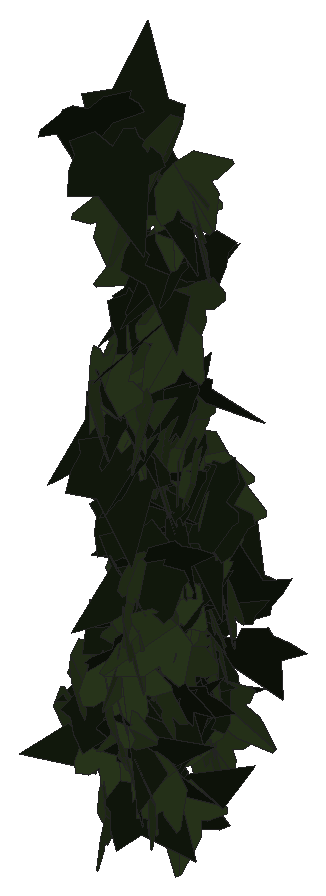
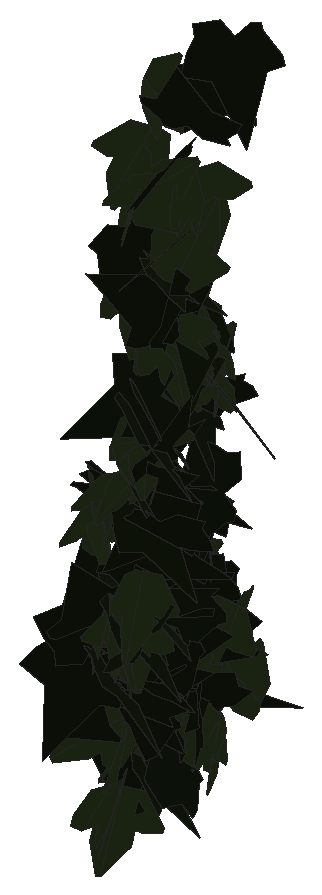
# SketchUp Ruby script. Lengths in inches.
U = 1.inch
M = Sketchup.active_model
def pt(a) = Geom::Point3d.new(a.map { |v| v * U })
def face(e, loops, mat)
  f = e.add_face(loops[0].map { |a| pt(a) })
  loops[1..].each { |l| e.add_face(l.map { |a| pt(a) }).erase! }
  f.material = f.back_material = mat if mat
  f
end
# faces: each face lists its corners as indices into pts; further lists are holes
def faces(e, pts, list, mat = nil) = list.each { |f| face(e, (f[0].is_a?(Array) ? f : [f]).map { |l| l.map { |i| pts[i] } }, mat) }
# xy, xz, yz: faces in a plane at the given z, y or x. An outline is a flat list of corners, or four numbers for a rectangle; further outlines are holes
def ring(l) = l.size == 4 ? [[l[0], l[1]], [l[2], l[1]], [l[2], l[3]], [l[0], l[3]]] : l.each_slice(2).to_a
def flat(e, list, mat, &to3) = list.each { |f| face(e, (f[0].is_a?(Array) ? f : [f]).map { |l| ring(l).map { |u, v| to3.(u, v) } }, mat) }
def xy(e, z, list, mat = nil) = flat(e, list, mat) { |x, y| [x, y, z] }
def xz(e, y, list, mat = nil) = flat(e, list, mat) { |x, z| [x, y, z] }
def yz(e, x, list, mat = nil) = flat(e, list, mat) { |y, z| [x, y, z] }
def lines(e, pts, list) = list.each { |a, b| e.add_line(pt(pts[a]), pt(pts[b])) }
# prism: a flat outline (further loops are holes) pulled along v
def prism(e, loops, v, mat = nil)
  f = face(e, loops, mat); d = Geom::Vector3d.new(v.map { |x| x * U })
  f.pushpull(f.normal.samedirection?(d) ? d.length : -d.length)
end
def box(e, o, s, mat = nil) = prism(e, [[o, [o[0] + s[0], o[1], o[2]], [o[0] + s[0], o[1] + s[1], o[2]], [o[0], o[1] + s[1], o[2]]]], [0, 0, s[2]], mat)
def at(x, y, z, deg = 0) = Geom::Transformation.translation(pt([x, y, z])) * Geom::Transformation.rotation(ORIGIN, Z_AXIS, deg.degrees)
def axes(o, x, y, z) = Geom::Transformation.new([*x, 0, *y, 0, *z, 0, *pt(o).to_a, 1])
def part(name) = M.definitions.add(name)
# library, detail: a bought-in or finely detailed component or shape, given as its bounding box
def library(name, o, s) = part(name).tap { |d| box(d.entities, o, s) }
def detail(e, o, s) = box(e.add_group.entities, o, s)
def put(e, d, t, mat = nil) = e.add_instance(d, t).tap { |i| i.material = mat if mat }
def group(e, t, mat = nil) = e.add_group.tap { |g| g.transformation = t; g.material = mat if mat }.entities
root = M.entities
M.materials.add("efeu1").color = [18, 25, 13]
M.materials.add("efeu2").color = [43, 57, 29]
c1 = part("ivyleaf_10")
p = [[0,0.5,-0.03],[-0.0625,2.02,-0.43],[-0.19,2.01,-0.46],[-0.54,1.05,-0.29],[-0.52,0.625,-0.18],[-0.83,0.76,-0.28],
  [-1.16,0.64,-0.33],[-1.15,0.33,-0.24],[-0.77,-0.39,0.02],[-0.3,-0.51,0.16],[0.04,-0.48,0.23],[-0.02,2.01,-0.4375],
  [-0.06,2.01,-0.43],[0.04,-0.49,0.23],[0.67,-0.49,0.14],[1.38,0.36,-0.2],[1.375,0.51,-0.24],[0.81,0.65,-0.19],
  [0.62,0.59,-0.15],[0.6,1.09,-0.28],[0.5,1.23,-0.31]]
faces(c1.entities,p,[[0,1,2,3,4,5,6,7,8,9,10],[11,12,0,13,14,15,16,17,18,19,20]],"efeu2")
c2 = part("ivyleaf_9")
p = [[1.54,2.16,1.25],[1.36,2.04,1.19],[-0.21,0.99,0.68],[-0.71,1.11,0.82],[-0.85,0.86,0.67],[-0.8,0.17,0.21],
  [-0.9,-0.01,0.1],[-0.67,-0.16,-0.02],[-0.08,-0.08,-0.05],[-0.03,-0.6,-0.4],[0.65,-0.88,-0.66],[0.83,-0.6,-0.49],
  [1.29,-0.42,-0.43],[1.8125,-0.07,-0.26],[1.21,0.44,0.15]]
faces(c2.entities,p,[[0,1,2,3,4,5,6,7,8,9,10,11,12,13,14]],"efeu1")
put(root,c1,axes([53,223.28,224.52],[-0.00386,0.01122,-0.49986],[0.44994,-0.21791,-0.00837],[-0.21803,-0.44988,-0.00841]))
put(root,c2,axes([52.83,223.04,233.82],[0.08421,0.46375,-0.16686],[-0.05301,-0.15977,-0.47081],[-0.49,0.09699,0.02226]))
put(root,c2,axes([53.08,223.25,233.2],[-0.19987,-0.25353,-0.3818],[0.29922,0.24332,-0.31821],[0.34716,-0.35569,0.05446]))
put(root,c1,axes([53.86,223.3,226.01],[0.30942,0.13896,-0.36736],[-0.35977,-0.08733,-0.33606],[-0.15756,0.4723,0.04595]))
put(root,c1,axes([53.24,223.1875,225.25],[0.43002,0.23566,0.09772],[0.08003,0.05724,-0.49022],[-0.24224,0.43725,0.01151]))
put(root,c1,axes([53.65,223.22,229.31],[0.28368,-0.39973,-0.09871],[-0.0436,0.09003,-0.48989],[0.40942,0.28656,0.01622]))
put(root,c1,axes([52.34,223.29,224.04],[-0.18407,-0.03169,0.4638],[0.4646,0.00496,0.18472],[-0.01631,0.49897,0.02762]))
put(root,c1,axes([53.18,223.55,225.48],[-0.05253,0.26045,-0.42356],[-0.01747,-0.42662,-0.26017],[-0.49693,-0.01253,0.05392]))
put(root,c1,axes([52.65,223.08,225.16],[-0.20071,0.42484,0.17096],[-0.07133,0.15538,-0.46986],[-0.45236,-0.213,-0.00176]))
put(root,c1,axes([53.12,223.02,223.1],[0.14543,-0.26559,-0.39789],[-0.08629,0.39448,-0.29486],[0.47053,0.15443,0.0689]))
put(root,c1,axes([53.4,223.23,226.11],[-0.18927,0.46048,-0.04623],[0.01831,-0.04245,-0.49786],[-0.46243,-0.19015,-0.00079]))
put(root,c2,axes([53.09,223.41,228.42],[-0.08934,-0.46202,-0.169],[0.04234,0.1639,-0.47047],[0.49013,-0.09837,0.00984]))
put(root,c1,axes([52.875,223.13,229.18],[-0.29879,0.35405,0.18807],[-0.13001,0.13631,-0.46316],[-0.37924,-0.32568,0.0106]))
put(root,c2,axes([53.6,223.58,226.86],[-0.4503,-0.17558,0.12806],[-0.11116,-0.06708,-0.48285],[0.18674,-0.46333,0.02138]))
put(root,c1,axes([53.47,223.49,226.75],[0.08,0.41052,-0.27399],[-0.05136,-0.26913,-0.41825],[-0.49088,0.09507,-0.0009]))
put(root,c1,axes([53.12,223.33,224.47],[-0.30037,0.39796,-0.03754],[-0.02457,0.02849,0.49858],[0.39897,0.30136,0.00244]))
put(root,c1,axes([53.8,223.1,223.55],[0.16888,-0.06911,-0.46552],[-0.24772,0.40747,-0.15036],[0.40014,0.28142,0.10338]))
put(root,c1,axes([53.04,223.37,224.05],[0.41823,0.26468,0.0709],[0.05836,0.04036,-0.49494],[-0.26773,0.42227,0.00286]))
put(root,c2,axes([53.15,223.33,223.93],[0.15139,-0.10012,0.4659],[0.46829,-0.05926,-0.1649],[0.08824,0.48628,0.07582]))
put(root,c2,axes([53.02,223.17,224.9],[-0.0163,-0.15179,-0.47612],[0.04488,0.47401,-0.15265],[0.49771,-0.04771,-0.00182]))
put(root,c1,axes([53.79,223.42,223.74],[0.38749,-0.04647,-0.31256],[-0.3036,0.08236,-0.38864],[0.08761,0.49097,0.03561]))
put(root,c1,axes([53.31,223.66,225.81],[-0.05468,-0.44399,0.22334],[-0.0218,-0.22233,-0.44732],[0.49652,-0.05865,0.00496]))
put(root,c2,axes([52.97,223.7,224.01],[-0.39964,-0.02866,0.29911],[-0.28524,-0.12029,-0.39264],[0.09447,-0.48447,0.0798]))
put(root,c1,axes([53.08,223.4375,224.43],[-0.19873,0.45755,-0.03404],[0.01356,-0.03122,-0.49884],[-0.45861,-0.19919,-0.00001]))
put(root,c2,axes([53.43,223.09,228.92],[0.04266,0.20923,0.45211],[0.01503,0.45302,-0.21107],[-0.49795,0.0316,0.03236]))
put(root,c2,axes([52.81,223.58,228.88],[-0.46289,0.1778,-0.06415],[0.05818,-0.02743,-0.49585],[-0.17985,-0.46651,0.00471]))
put(root,c2,axes([53.4,223.27,228.33],[-0.1798,0.43169,0.17696],[-0.07297,0.16129,-0.46761],[-0.46081,-0.19398,0.005]))
put(root,c2,axes([53.1875,223.17,225.63],[0.20786,0.4302,0.14738],[0.07592,0.12694,-0.47762],[-0.44836,0.22093,-0.01255]))
put(root,c1,axes([53.49,223.64,226.67],[0.08357,0.45729,-0.18414],[-0.02902,-0.18188,-0.46484],[-0.49211,0.08838,-0.00386]))
put(root,c2,axes([53.5,223.84,224.49],[-0.14694,-0.47564,0.04667],[-0.01523,-0.04414,-0.49781],[0.47768,-0.14771,-0.00152]))
put(root,c1,axes([53.07,223.62,226.63],[0.40653,-0.28992,-0.02608],[-0.02147,0.0148,-0.49932],[0.2903,0.4071,-0.00042]))
put(root,c1,axes([52.78,223.68,228.97],[0.38678,0.03452,0.31498],[0.31396,0.02532,-0.38831],[-0.04276,0.49816,-0.00209]))
put(root,c2,axes([52.8125,223.86,223.88],[0.00967,-0.04163,-0.49817],[0.49243,-0.08508,0.01667],[-0.08616,-0.49095,0.03935]))
put(root,c1,axes([52.68,223.63,229.23],[0.47989,-0.13412,-0.0414],[0.04517,0.00793,0.49789],[-0.13289,-0.48161,0.01973]))
put(root,c1,axes([53.54,223.82,225.8],[0.40671,-0.27336,0.09932],[0.07891,-0.06062,-0.49],[0.27993,0.41424,-0.00617]))
put(root,c2,axes([53.34,223.53,223.41],[0.07491,-0.27222,-0.41266],[-0.12722,0.3927,-0.28214],[0.47771,0.14727,-0.01043]))
put(root,c1,axes([52.71,223.61,225.2],[-0.41738,-0.20417,-0.1847],[0.15937,0.09435,-0.46443],[0.2245,-0.44656,-0.01368]))
put(root,c1,axes([53.47,223.98,233.27],[0.12526,-0.39446,0.28056],[0.0925,-0.26495,-0.41382],[0.47514,0.15557,0.0066]))
put(root,c2,axes([52.9,223.59,226.65],[0.43487,-0.13092,-0.20915],[-0.19039,0.09155,-0.45318],[0.15696,0.47379,0.02978]))
put(root,c1,axes([53.46,223.68,224.91],[-0.46229,0.19016,-0.0111],[0.00921,-0.0068,-0.49987],[-0.19027,-0.46238,0.00278]))
put(root,c2,axes([52.67,224,228.89],[0.21166,-0.40767,0.1975],[0.11969,-0.15992,-0.45837],[0.4369,0.24131,0.02989]))
put(root,c2,axes([53.46,223.51,226.95],[0.32519,0.37964,0.01141],[0.00754,0.00856,-0.49987],[-0.37973,0.32527,-0.00015]))
put(root,c1,axes([52.92,223.48,223.27],[0.00985,0.30233,0.39812],[-0.11217,0.38938,-0.29292],[-0.48716,-0.08354,0.0755]))
put(root,c2,axes([53.54,223.65,225.07],[0.42366,0.15824,-0.21324],[-0.20643,-0.05627,-0.45191],[-0.16702,0.47095,0.01766]))
put(root,c1,axes([52.7,223.94,231.99],[-0.20095,-0.44771,0.0958],[0.00584,-0.10712,-0.48835],[0.45781,-0.19515,0.04828]))
put(root,c1,axes([53.67,223.86,225.33],[-0.35644,-0.35063,-0.00302],[-0.0001,0.0044,-0.49998],[0.35064,-0.35643,-0.00321]))
put(root,c2,axes([52.91,223.94,225.78],[-0.10934,-0.4117,-0.26182],[0.11484,0.23906,-0.42386],[0.47419,-0.15282,0.04228]))
put(root,c2,axes([53.03,223.99,223.46],[0.23736,-0.20265,0.39063],[0.33445,-0.20539,-0.30977],[0.28601,0.40835,0.03805]))
put(root,c2,axes([53.01,224.24,224.98],[-0.01527,-0.13647,-0.48077],[-0.06019,-0.477,0.13731],[-0.49613,0.06207,-0.00186]))
put(root,c2,axes([52.99,223.65,229.88],[0.00908,0.4782,0.14573],[-0.05682,0.1458,-0.47488],[-0.49668,-0.00794,0.05699]))
put(root,c1,axes([53.37,224.17,226.1],[0.18449,0.36276,-0.29046],[-0.13769,-0.25581,-0.40694],[-0.44385,0.23015,0.00551]))
put(root,c1,axes([53.26,224.05,228.46],[0.00271,-0.4975,-0.04989],[0.00659,0.04993,-0.49746],[0.49995,0.00204,0.00682]))
put(root,c1,axes([53.47,224.11,230.11],[0.47024,-0.03701,-0.16585],[-0.16512,0.01579,-0.47168],[0.04015,0.49838,0.00263]))
put(root,c1,axes([52.74,224.32,230.9375],[-0.24552,-0.32435,-0.29072],[-0.17646,-0.23104,0.4068],[-0.39822,0.30235,-0.00101]))
put(root,c2,axes([52.8,224.0625,227.33],[-0.11752,-0.23267,-0.42668],[0.283,0.3241,-0.25469],[0.39509,-0.30136,0.05552]))
put(root,c2,axes([52.74,223.76,225.57],[0.33248,0.05183,0.36982],[0.2932,0.27043,-0.3015],[-0.23127,0.41735,0.14943]))
put(root,c2,axes([52.36,223.97,227.38],[0.40154,-0.0909,0.28373],[0.29375,0.04126,-0.4025],[0.04976,0.48993,0.08654]))
put(root,c1,axes([53.55,224.11,223.02],[0.16134,0.46945,-0.05988],[-0.02775,-0.05378,-0.49632],[-0.47244,0.16348,0.0087]))
put(root,c2,axes([53.18,223.74,224.59],[0.16763,0.16788,0.44013],[0.17398,0.41207,-0.22344],[-0.43776,0.22806,0.07973]))
put(root,c1,axes([52.99,223.89,224.9],[-0.11227,0.36592,0.32171],[-0.21751,0.25778,-0.36911],[-0.43599,-0.22283,0.1013]))
put(root,c1,axes([53.2,224.0625,227.98],[-0.31515,0.38748,0.02331],[-0.01469,0.01809,-0.49946],[-0.3879,-0.31549,-0.00001]))
put(root,c2,axes([53.45,223.99,224.6],[0.32287,0.35293,-0.14559],[-0.09192,-0.1132,-0.47826],[-0.37055,0.3356,-0.00821]))
put(root,c2,axes([53.14,224.42,230.91],[-0.44715,0.09183,-0.20401],[0.15086,-0.21292,-0.4265],[-0.16521,-0.44298,0.16271]))
put(root,c2,axes([53,224.44,231.05],[0.06112,-0.49022,0.07715],[0.07388,-0.06788,-0.48983],[0.49072,0.07128,0.06414]))
put(root,c1,axes([53.17,224.07,223.55],[0.19963,0.42782,0.16466],[0.06452,0.15159,-0.47208],[-0.45386,0.20973,0.00531]))
put(root,c1,axes([53.67,223.97,228.28],[-0.03531,0.22818,0.44349],[-0.37216,0.28394,-0.17572],[-0.33204,-0.34251,0.14979]))
put(root,c2,axes([53.53,223.88,224.39],[0.13588,0.42884,0.21825],[0.06676,0.20779,-0.44985],[-0.47653,0.15139,-0.00079]))
put(root,c1,axes([52.93,224.35,229.8],[-0.20883,-0.44797,0.07559],[-0.03399,-0.06755,-0.49425],[0.45303,-0.21157,-0.00224]))
put(root,c1,axes([52.92,224.39,229.81],[0.29847,0.28086,-0.28641],[-0.26393,-0.13134,-0.40384],[-0.30208,0.39226,0.06986]))
put(root,c2,axes([52.77,224.125,233.04],[-0.47139,0.03572,0.16285],[0.16254,-0.01022,0.47273],[0.0371,0.49862,-0.00197]))
put(root,c2,axes([53.67,224.0625,223.65],[-0.15528,0.44039,0.17874],[-0.08777,0.15823,-0.46611],[-0.4671,-0.17613,0.02817]))
put(root,c2,axes([52.98,224.39,232.34],[0.20105,-0.44219,-0.11854],[-0.04461,0.10993,-0.48572],[0.45562,0.20588,0.00475]))
put(root,c2,axes([52.86,224.17,229.93],[-0.13914,-0.2767,0.39252],[0.17292,0.35239,0.30971],[-0.44804,0.22194,-0.00237]))
put(root,c2,axes([53.41,224.54,231.35],[-0.01358,0.20407,-0.45626],[-0.00974,-0.45645,-0.20386],[-0.49972,0.00335,0.01637]))
put(root,c1,axes([53.34,224.46,231.89],[-0.32069,0.03088,-0.38237],[-0.38219,-0.06854,0.31501],[-0.03296,0.49432,0.06757]))
put(root,c1,axes([52.93,224.52,224.53],[0.40418,-0.2021,0.21401],[0.19059,-0.09736,-0.45188],[0.22432,0.44685,-0.00166]))
put(root,c1,axes([53.18,224.35,232.05],[0.26293,0.42521,0.00788],[0.00379,0.00692,-0.49994],[-0.42527,0.26295,0.00041]))
put(root,c1,axes([53.53,224.17,232.52],[0.19103,0.39448,0.2406],[-0.00304,0.26142,-0.42621],[-0.46206,0.16138,0.10228]))
put(root,c2,axes([52.93,224.0625,226.64],[0.23883,0.41164,0.15333],[0.07878,0.13156,-0.4759],[-0.43215,0.25148,-0.00202]))
put(root,c2,axes([53.25,224.36,222.71],[-0.0141,-0.10907,0.48775],[0.49656,-0.05855,0.00126],[0.05684,0.48443,0.10998]))
put(root,c2,axes([52.9375,224.69,224.46],[-0.17547,-0.46814,0.0077],[-0.00276,-0.00719,-0.49994],[0.46819,-0.17549,-0.00006]))
put(root,c2,axes([53.24,224.62,228.98],[-0.42298,0.16305,-0.21096],[0.19324,-0.08511,-0.45323],[-0.18371,-0.46494,0.00899]))
put(root,c1,axes([53.35,224.5,230.49],[-0.24176,-0.43471,-0.05079],[0.02909,0.04193,-0.49739],[0.4367,-0.24345,0.00502]))
put(root,c2,axes([52.8,224.33,225.1],[0.49039,0.09285,0.02991],[0.02947,0.00513,-0.4991],[-0.09299,0.49128,-0.00045]))
put(root,c2,axes([53.21,224.27,225.39],[-0.088,0.34432,0.35171],[-0.26987,0.26504,-0.32699],[-0.41161,-0.24739,0.13919]))
put(root,c2,axes([53.33,224.73,227.01],[0.16746,-0.46965,0.0372],[0.02097,-0.03201,-0.49853],[0.47066,0.16853,0.00898]))
put(root,c2,axes([53.1,224.82,227.71],[-0.43717,-0.2155,0.11156],[-0.09489,-0.05975,-0.48726],[0.22334,-0.4472,0.01134]))
put(root,c1,axes([53.42,224.55,231.87],[-0.29728,0.38309,-0.12193],[0.07335,-0.09742,-0.4849],[-0.39528,-0.30619,0.00172]))
put(root,c2,axes([53.84,224.79,227.35],[-0.46852,-0.05848,0.16452],[-0.1548,-0.07883,-0.46885],[0.08078,-0.49027,0.05576]))
put(root,c2,axes([53.82,224.66,227.44],[-0.46966,0.14031,0.09867],[-0.10758,-0.01694,-0.488],[-0.13359,-0.47961,0.0461]))
put(root,c2,axes([52.86,224.17,223.12],[0.11228,0.31341,0.37306],[0.04645,0.3742,-0.32835],[-0.48501,0.10839,0.05491]))
put(root,c2,axes([53.0625,224.72,223.32],[-0.3923,0.20417,-0.23327],[0.18067,-0.15515,-0.43964],[-0.25191,-0.42924,0.04796]))
put(root,c2,axes([53.61,224.46,225.875],[-0.22927,0.42664,0.12416],[-0.12201,0.07389,-0.47922],[-0.42726,-0.25004,0.07023]))
put(root,c2,axes([52.81,224.4,230.2],[0.0061,-0.02122,0.49951],[0.45316,0.21127,0.00344],[-0.21121,0.45267,0.02181]))
put(root,c2,axes([53.16,224.94,226.66],[-0.07468,-0.12697,-0.47781],[-0.22427,-0.42195,0.14718],[-0.4406,0.2363,0.00607]))
put(root,c2,axes([52.74,224.34,227.3125],[0.30813,0.33779,0.20237],[0.14747,0.13928,-0.45701],[-0.36511,0.34132,-0.01379]))
put(root,c2,axes([53.29,224.75,227.69],[-0.4305,0.22343,-0.12145],[0.11141,-0.04896,-0.48497],[-0.2286,-0.44462,-0.00763]))
put(root,c2,axes([52.875,224.68,227.98],[-0.16681,-0.41229,0.22846],[0.08448,0.21227,0.44475],[-0.46372,0.18697,-0.00116]))
put(root,c1,axes([52.99,224.78,228.55],[-0.22129,-0.44719,-0.03238],[0.03144,0.02054,-0.49859],[0.44726,-0.2227,0.01903]))
put(root,c2,axes([53.17,225.02,224.3125],[-0.42796,-0.25829,-0.01163],[0.01034,0.00538,-0.49986],[0.25834,-0.42809,0.00074]))
put(root,c2,axes([52.61,224.94,227.25],[-0.18377,-0.35355,-0.30204],[0.1936,0.23712,-0.39534],[0.42279,-0.26225,0.04974]))
put(root,c2,axes([53.15,224.84,228.78],[-0.3925,0.30903,-0.02111],[0.01088,-0.0203,-0.49947],[-0.30956,-0.39254,0.00922]))
put(root,c2,axes([52.87,224.68,229.02],[0.47218,0.00991,0.16417],[0.16114,0.07193,-0.46782],[-0.03288,0.4947,0.06473]))
put(root,c2,axes([52.97,225.06,224.61],[-0.27574,-0.35075,-0.2257],[0.18745,0.13749,-0.44267],[0.3726,-0.32874,0.05568]))
put(root,c2,axes([53.02,224.85,227.27],[-0.24262,0.4259,-0.09874],[-0.0564,-0.14247,-0.47594],[-0.43354,-0.21981,0.11717]))
put(root,c1,axes([53.2,225.08,225.02],[0.23832,-0.15013,0.41312],[0.38314,-0.15937,-0.27894],[0.21543,0.44951,0.03908]))
put(root,c2,axes([52.96,224.55,224.15],[0.29375,0.19303,0.3556],[0.26699,0.2377,-0.34959],[-0.30402,0.39527,0.03657]))
put(root,c1,axes([53.33,224.67,227.55],[0.08061,-0.29966,-0.39205],[0.02338,0.39912,-0.30026],[0.49291,0.03008,0.07835]))
put(root,c1,axes([53.36,224.9,227.6],[0.15116,0.47658,-0.00435],[-0.01387,-0.00016,-0.49981],[-0.4764,0.15122,0.01317]))
put(root,c1,axes([53.57,225.04,227.1875],[0.07299,0.48351,-0.10435],[-0.01532,-0.10322,-0.48899],[-0.49441,0.07458,-0.00025]))
put(root,c2,axes([52.67,225.23,225.61],[0.18843,-0.39147,0.24748],[0.20779,-0.16732,-0.42288],[0.4139,0.26222,0.09963]))
put(root,c1,axes([53.41,225.15,226.75],[0.23729,-0.41093,-0.15757],[0.08207,-0.13455,0.47451],[-0.43239,-0.25105,0.0036]))
put(root,c2,axes([53.15,225.04,225.77],[-0.34075,0.35885,-0.07153],[0.01572,-0.0833,-0.49276],[-0.36557,-0.33807,0.04549]))
put(root,c1,axes([53.21,225.1,225.37],[-0.35587,0.34016,-0.08745],[0.06936,-0.05398,-0.49221],[-0.34431,-0.36246,-0.00877]))
put(root,c1,axes([53.03,224.79,227.92],[-0.00555,0.22419,0.44688],[-0.06355,0.44297,-0.22302],[-0.49591,-0.05927,0.02358]))
put(root,c2,axes([53.45,225.34,225.34],[0.3263,0.27803,0.25735],[-0.21393,-0.14509,0.428],[0.31267,-0.38942,0.02427]))
put(root,c2,axes([53.32,225.16,224.87],[-0.32728,0.36612,0.09406],[-0.0757,0.05842,-0.49077],[-0.37035,-0.33548,0.01719]))
put(root,c1,axes([53.4,225.22,225.84],[-0.39424,0.30603,0.03031],[-0.0486,-0.01335,-0.49745],[-0.30366,-0.39518,0.04027]))
put(root,c1,axes([52.87,225.3,225.66],[0.45023,0.21596,-0.02562],[-0.04301,0.03068,-0.4972],[-0.21318,0.44991,0.0462]))
put(root,c1,axes([53.29,225.18,223.98],[0.30566,0.00292,0.39568],[0.3365,0.26114,-0.26187],[-0.20819,0.42638,0.15767]))
put(root,c1,axes([52.65,225.29,226.35],[-0.11153,-0.44003,-0.20961],[0.04602,0.20456,-0.45391],[0.48522,-0.12054,-0.00513]))
put(root,c2,axes([53.49,225.25,225.53],[-0.25781,-0.20288,0.37732],[0.29628,0.23365,0.32807],[-0.30944,0.39275,-0.00026]))
put(root,c2,axes([53.58,225.32,224.9375],[0.38925,0.30311,-0.0813],[-0.0536,-0.06341,-0.49306],[-0.30921,0.39256,-0.01687]))
put(root,c1,axes([52.84,225.53,223.93],[-0.22963,0.43957,-0.06361],[0.00161,-0.07079,-0.49496],[-0.44415,-0.22752,0.03109]))
put(root,c1,axes([52.82,225.61,223.1],[-0.34671,-0.34462,-0.10502],[0.09846,0.04956,-0.4877],[0.34655,-0.35886,0.0335]))
put(root,c1,axes([52.83,225.64,223.3],[-0.13825,0.47954,0.03043],[-0.00652,0.02978,-0.49907],[-0.48046,-0.13839,-0.00198]))
